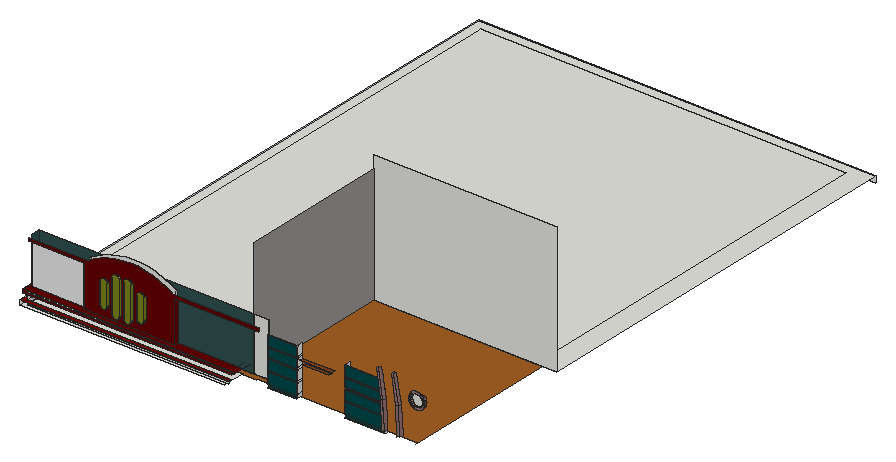
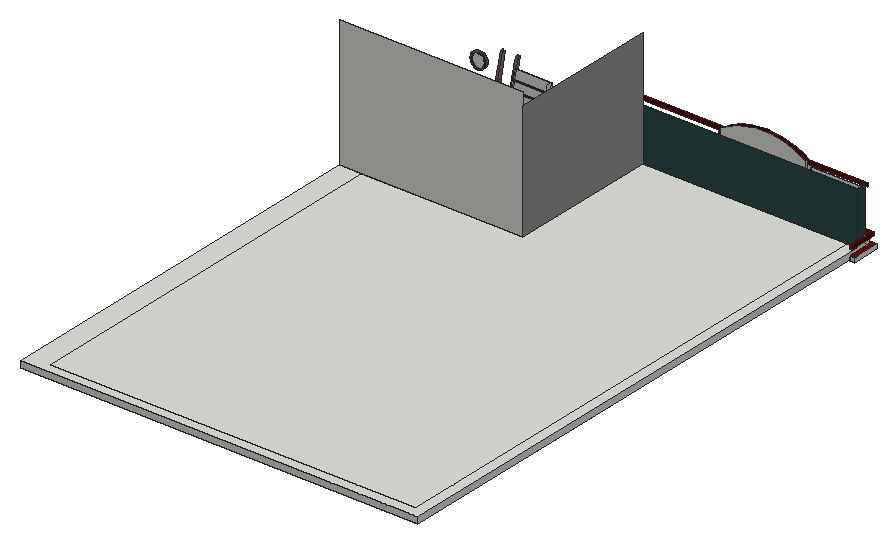
# SketchUp Ruby script. Lengths in inches.
U = 1.inch
M = Sketchup.active_model
def pt(a) = Geom::Point3d.new(a.map { |v| v * U })
def face(e, loops, mat)
  f = e.add_face(loops[0].map { |a| pt(a) })
  loops[1..].each { |l| e.add_face(l.map { |a| pt(a) }).erase! }
  f.material = f.back_material = mat if mat
  f
end
# faces: each face lists its corners as indices into pts; further lists are holes
def faces(e, pts, list, mat = nil) = list.each { |f| face(e, (f[0].is_a?(Array) ? f : [f]).map { |l| l.map { |i| pts[i] } }, mat) }
# xy, xz, yz: faces in a plane at the given z, y or x. An outline is a flat list of corners, or four numbers for a rectangle; further outlines are holes
def ring(l) = l.size == 4 ? [[l[0], l[1]], [l[2], l[1]], [l[2], l[3]], [l[0], l[3]]] : l.each_slice(2).to_a
def flat(e, list, mat, &to3) = list.each { |f| face(e, (f[0].is_a?(Array) ? f : [f]).map { |l| ring(l).map { |u, v| to3.(u, v) } }, mat) }
def xy(e, z, list, mat = nil) = flat(e, list, mat) { |x, y| [x, y, z] }
def xz(e, y, list, mat = nil) = flat(e, list, mat) { |x, z| [x, y, z] }
def yz(e, x, list, mat = nil) = flat(e, list, mat) { |y, z| [x, y, z] }
def lines(e, pts, list) = list.each { |a, b| e.add_line(pt(pts[a]), pt(pts[b])) }
# prism: a flat outline (further loops are holes) pulled along v
def prism(e, loops, v, mat = nil)
  f = face(e, loops, mat); d = Geom::Vector3d.new(v.map { |x| x * U })
  f.pushpull(f.normal.samedirection?(d) ? d.length : -d.length)
end
def box(e, o, s, mat = nil) = prism(e, [[o, [o[0] + s[0], o[1], o[2]], [o[0] + s[0], o[1] + s[1], o[2]], [o[0], o[1] + s[1], o[2]]]], [0, 0, s[2]], mat)
def at(x, y, z, deg = 0) = Geom::Transformation.translation(pt([x, y, z])) * Geom::Transformation.rotation(ORIGIN, Z_AXIS, deg.degrees)
def axes(o, x, y, z) = Geom::Transformation.new([*x, 0, *y, 0, *z, 0, *pt(o).to_a, 1])
def part(name) = M.definitions.add(name)
# library, detail: a bought-in or finely detailed component or shape, given as its bounding box
def library(name, o, s) = part(name).tap { |d| box(d.entities, o, s) }
def detail(e, o, s) = box(e.add_group.entities, o, s)
def put(e, d, t, mat = nil) = e.add_instance(d, t).tap { |i| i.material = mat if mat }
def group(e, t, mat = nil) = e.add_group.tap { |g| g.transformation = t; g.material = mat if mat }.entities
root = M.entities
M.materials.add("[0001_PaleVioletRed]").color = [219, 112, 147]
M.materials.add("[0022_Maroon]").color = [99, 0, 0]
M.materials.add("[0022_Maroon]1").color = [128, 0, 0]
M.materials.add("[0043_SaddleBrown]").color = [139, 69, 19]
M.materials.add("[0057_DarkKhaki]").color = [122, 132, 27]
M.materials.add("[0078_DarkSlateGray]").color = [47, 79, 79]
M.materials.add("[0119_RosyBrown]").color = [150, 114, 114]
M.materials.add("[Color H08]").color = [0, 71, 71]
M.materials.add("[Concrete Aggregate Smoke]").color = [154, 150, 148]
M.materials.add("[Polished Concrete Old]").color = [229, 229, 229]
M.materials.add("[Wood Square Tile 02]").color = [160, 95, 34]
xy(root,244.39,[[2.625,634.61,2.625,660.18,7.28,660.18,7.28,637.61,193.58,637.61,193.58,634.61]])
xy(root,245.03,[[221.0625,650.11,247.97,651.11],[292.45,650.11,328.99,651.11]],"[Color H08]")
xy(root,245.51,[[7,637.61,7.28,654.03],[7.28,637.61,194.39,654.03],[7,654.03,7.28,654.11],[7,654.11,7.28,660.18],[7.28,654.11,29.57,654.11,29.57,663.11,7,663.11,7,660.18,7.28,660.18],
  [[71.2,714.73,131.64,714.73,131.64,851.92,121.29,851.92,121.29,841.18,126.31,841.18,126.31,725.47,76.53,725.47,76.53,779.39,114.56,779.39,114.56,851.92,71.2,851.92],[76.53,788.7,109.94,841.18]],[7,756.4375,11.62,787.78],[11.62,756.4375,16,787.78],[7,927.36,358,927.36,358,933.36,16,933.36,16,1154.11,358,1154.11,358,1163.11,7,1163.11]])
xy(root,245.51,[[[25.34,691.07,164.1,890.37],[71.2,714.73,131.64,714.73,131.64,851.92,121.29,851.92,121.29,841.18,126.31,841.18,126.31,725.47,76.53,725.47,76.53,779.39,114.56,779.39,114.56,851.92,71.2,851.92]],[76.53,788.7,109.94,841.18]],"[0057_DarkKhaki]")
xy(root,245.51,[[[7.28,654.03,7.28,654.11,29.57,654.11,29.57,663.11,7,663.11,7,1163.11,358,1163.11,358,654.11,207.9375,654.11,207.9375,654.03],[11.62,663.42,177.82,918.03]]],"[Wood Square Tile 02]")
xy(root,247.73,[[221.0625,650.11,247.97,651.11],[292.45,650.11,329.17,651.11]],"[Color H08]")
xy(root,247.85,[[[11.62,663.42,177.82,918.03],[25.34,691.07,164.1,890.37]]],"[0001_PaleVioletRed]")
xy(root,248.7,[[2.625,634.61,197.0625,634.61,197.0625,637.61,7,637.61,7,660.18,2.625,660.18]],"[0022_Maroon]1")
xy(root,251.36,[[207.9375,651.11,221.0625,651.24],[7,651.24,16,651.24,16,1154.11,358,1154.11,358,791.05,377.9375,791.05,377.9375,1163.11,7,1163.11],[16,651.24,207,651.24,207,791.05,358,791.05,358,1154.11,16,1154.11]])
xy(root,254.68,[[4.6875,634.61,4.6875,660.18,7,660.18,7,637.61,200.08,637.61,200.08,634.61]],"[0022_Maroon]")
xy(root,258.06,[[57.84,639.11,143.09,640.93],[57.84,640.93,57.84,642.11,61.4,642.11,61.4,643.36,141.15,643.36,141.15,642.11,143.09,642.11,143.09,640.93]])
xy(root,258.06,[[4.6875,634.61,203.6875,634.61,203.6875,642.11,143.09,642.11,143.09,639.11,57.84,639.11,57.84,642.11,7,642.11,7,660.18,4.6875,660.18]],"[0022_Maroon]")
xy(root,258.11,[[221.0625,650.11,247.97,651.11],[292.45,650.11,328.77,651.11]],"[Color H08]")
xy(root,259.56,[[221.0625,650.11,247.97,651.11],[292.45,650.11,328.72,651.11]],"[Color H08]")
xy(root,268.56,[[221.0625,650.11,247.97,651.11],[292.45,650.11,328.375,651.11]],"[Color H08]")
xy(root,270.44,[[221.0625,650.11,247.97,651.11],[292.45,650.11,328.3,651.11]],"[Color H08]")
xy(root,278.01,[[221.0625,650.11,247.97,651.11],[292.45,650.11,327.36,651.11]],"[Color H08]")
xy(root,278.93,[[258.01,645.11,281.88,648.11]],"[0043_SaddleBrown]")
xy(root,279.73,[[221.0625,650.11,247.97,651.11],[292.45,650.11,327.07,651.11]],"[Color H08]")
xy(root,281.93,[[255.01,645.11,284.88,648.11]],"[0043_SaddleBrown]")
xz(root,637.11,[[89.45,261.33,90.33,261.4375,91.15,261.74,91.89,262.23,92.49,262.875,92.93,263.64,93.17,264.49,93.17,295.18,92.89,295.99,92.44,296.72,91.84,297.33,91.12,297.79,90.31,298.08,89.45,298.18,88.6,298.08,87.79,297.79,87.0625,297.33,86.46,296.72,86.01,295.99,85.73,295.18,85.73,264.49,85.98,263.64,86.41,262.875,87.01,262.23,87.75,261.74,88.58,261.4375],[100.39,261.33,101.26,261.4375,102.09,261.74,102.83,262.23,103.43,262.875,103.86,263.64,104.11,264.49,104.11,295.18,103.83,295.99,103.38,296.72,102.78,297.33,102.05,297.79,101.24,298.08,100.39,298.18,99.54,298.08,98.73,297.79,98,297.33,97.4,296.72,96.95,295.99,96.67,295.18,96.67,264.49,96.91,263.64,97.35,262.875,97.95,262.23,98.6875,261.74,99.51,261.4375],[78.26,265.89,79.12,266.01,79.92,266.34,80.6,266.86,81.13,267.55,81.46,268.35,81.57,269.21,81.57,288.64,81.27,289.31,80.85,289.9,80.31,290.38,79.67,290.75,78.98,290.97,78.26,291.05,77.54,290.97,76.84,290.75,76.21,290.38,75.67,289.9,75.24,289.31,74.95,288.64,74.95,269.21,75.06,268.35,75.39,267.55,75.92,266.86,76.6,266.34,77.4,266.01],[112.38,265.89,113.24,266.01,114.04,266.34,114.73,266.86,115.25,267.55,115.58,268.35,115.7,269.21,115.7,288.64,115.4,289.31,114.97,289.9,114.43,290.38,113.8,290.75,113.11,290.97,112.38,291.05,111.66,290.97,110.97,290.75,110.34,290.38,109.8,289.9,109.37,289.31,109.07,288.64,109.07,269.21,109.18,268.35,109.52,267.55,110.04,266.86,110.73,266.34,111.53,266.01]],"[0057_DarkKhaki]")
xz(root,637.61,[[7.28,244.39,194.39,245.51],[7,245.51,7.28,248.7]])
xz(root,639.11,[[[57.84,258.06,143.09,258.06,143.09,296.25,221.0625,296.25,221.0625,299.9,140.36,299.9,140.36,300.29,134.72,303.6,128.42,306.52,121.85,308.82,115.1,310.48,108.22,311.49,101.28,311.82,94.33,311.49,87.45,310.48,80.7,308.82,74.14,306.52,67.83,303.6,61.62,299.95,7,299.95,7,296.97,57.84,296.97],[89.45,261.33,88.58,261.4375,87.75,261.74,87.01,262.23,86.41,262.875,85.98,263.64,85.73,264.49,85.73,295.18,86.01,295.99,86.46,296.72,87.0625,297.33,87.79,297.79,88.6,298.08,89.45,298.18,90.31,298.08,91.12,297.79,91.84,297.33,92.44,296.72,92.89,295.99,93.17,295.18,93.17,264.49,92.93,263.64,92.49,262.875,91.89,262.23,91.15,261.74,90.33,261.4375],[100.39,261.33,99.51,261.4375,98.6875,261.74,97.95,262.23,97.35,262.875,96.91,263.64,96.67,264.49,96.67,295.18,96.95,295.99,97.4,296.72,98,297.33,98.73,297.79,99.54,298.08,100.39,298.18,101.24,298.08,102.05,297.79,102.78,297.33,103.38,296.72,103.83,295.99,104.11,295.18,104.11,264.49,103.86,263.64,103.43,262.875,102.83,262.23,102.09,261.74,101.26,261.4375],[78.26,265.89,77.4,266.01,76.6,266.34,75.92,266.86,75.39,267.55,75.06,268.35,74.95,269.21,74.95,288.64,75.24,289.31,75.67,289.9,76.21,290.38,76.84,290.75,77.54,290.97,78.26,291.05,78.98,290.97,79.67,290.75,80.31,290.38,80.85,289.9,81.27,289.31,81.57,288.64,81.57,269.21,81.46,268.35,81.13,267.55,80.6,266.86,79.92,266.34,79.12,266.01],[112.38,265.89,111.53,266.01,110.73,266.34,110.04,266.86,109.52,267.55,109.18,268.35,109.07,269.21,109.07,288.64,109.37,289.31,109.8,289.9,110.34,290.38,110.97,290.75,111.66,290.97,112.38,291.05,113.11,290.97,113.8,290.75,114.43,290.38,114.97,289.9,115.4,289.31,115.7,288.64,115.7,269.21,115.58,268.35,115.25,267.55,114.73,266.86,114.04,266.34,113.24,266.01]]],"[0022_Maroon]")
xz(root,642.11,[[57.84,258.06,61.4,298.09],[141.15,258.06,143.09,296.25]])
xz(root,642.11,[[7,258.06,57.84,296.97]],"[Polished Concrete Old]")
xz(root,643.36,[[61.4,258.06,61.4,300.74,67.46,304.29,73.84,307.25,80.47,309.58,87.3,311.26,94.26,312.27,101.28,312.61,108.3,312.27,115.25,311.26,122.08,309.58,128.71,307.25,135.09,304.29,141.15,300.74,141.15,258.06]])
xz(root,649.11,[[[360.63,275.86,362.59,276.11,364.42,276.87,365.98,278.07,367.18,279.64,367.94,281.46,368.2,283.42,367.94,285.375,367.18,287.2,365.98,288.77,364.42,289.97,362.59,290.72,360.63,290.98,358.68,290.72,356.85,289.97,355.29,288.77,354.09,287.2,353.33,285.375,353.07,283.42,353.33,281.46,354.09,279.64,355.29,278.07,356.85,276.87,358.68,276.11],[360.63,277.52,359.11,277.72,357.6875,278.3125,356.47,279.25,355.53,280.47,354.94,281.89,354.74,283.42,354.94,284.94,355.53,286.37,356.47,287.59,357.6875,288.52,359.11,289.11,360.63,289.3125,362.16,289.11,363.58,288.52,364.8,287.59,365.74,286.37,366.33,284.94,366.53,283.42,366.33,281.89,365.74,280.47,364.8,279.25,363.58,278.3125,362.16,277.72]]],"[0119_RosyBrown]")
xz(root,650.11,[[221.0625,247.73,247.97,258.11],[292.45,247.73,329.17,247.73,328.77,258.11,292.45,258.11],[221.0625,259.56,247.97,268.56],[292.45,259.56,328.72,259.56,328.375,268.56,292.45,268.56],[221.0625,270.44,247.97,278.01],
  [292.45,270.44,328.3,270.44,328.2,273.08,327.36,278.01,292.45,278.01],[221.0625,279.73,247.97,288.67],[292.45,279.73,327.07,279.73,325.55,288.67,292.45,288.67]],"[Color H08]")
xz(root,651.11,[[328.99,245.03,331.29,245.03,331.5,247.73,329.17,247.73,329.19,247.23],[221.0625,247.73,247.97,258.11],[292.45,247.73,292.45,258.11,328.77,258.11,329.17,247.73],[329.17,247.73,331.5,247.73,331.53,248.09,331.03,258.11,328.77,258.11],[328.77,258.11,331.03,258.11,330.96,259.56,328.72,259.56],
  [221.0625,259.56,247.97,268.56],[292.45,259.56,292.45,268.56,328.375,268.56,328.72,259.56],[328.72,259.56,330.96,259.56,330.5,268.56,328.375,268.56],[328.375,268.56,330.5,268.56,330.41,270.44,328.3,270.44],[221.0625,270.44,247.97,278.01],
  [292.45,270.44,292.45,278.01,327.36,278.01,328.2,273.08,328.3,270.44],[328.3,270.44,330.41,270.44,330.25,273.68,329.47,278.01,327.36,278.01,328.2,273.08],[360.63,277.52,362.16,277.72,363.58,278.3125,364.8,279.25,365.74,280.47,366.33,281.89,366.53,283.42,366.33,284.94,365.74,286.37,364.8,287.59,363.58,288.52,362.16,289.11,360.63,289.3125,359.11,289.11,357.6875,288.52,356.47,287.59,355.53,286.37,354.94,284.94,354.74,283.42,354.94,281.89,355.53,280.47,356.47,279.25,357.6875,278.3125,359.11,277.72],[327.36,278.01,329.47,278.01,329.16,279.73,327.07,279.73],[221.0625,279.73,247.97,288.67],
  [292.45,279.73,292.45,288.67,325.55,288.67,327.07,279.73],[327.07,279.73,329.16,279.73,327.54,288.67,325.55,288.67]])
xz(root,651.11,[[221.0625,245.03,247.97,247.73],[292.45,245.03,328.99,245.03,329.19,247.23,329.17,247.73,292.45,247.73],[221.0625,258.11,247.97,259.56],[292.45,258.11,328.77,258.11,328.72,259.56,292.45,259.56],[221.0625,268.56,247.97,270.44],
  [292.45,268.56,328.375,268.56,328.3,270.44,292.45,270.44],[221.0625,278.01,247.97,279.73],[292.45,278.01,327.36,278.01,327.07,279.73,292.45,279.73]],"[Color H08]")
xz(root,651.24,[[207,251.36,221.0625,300.74]])
xz(root,651.24,[[7,251.36,207,300.74]],"[0078_DarkSlateGray]")
xz(root,660.18,[[2.625,244.39,2.625,248.7,7,248.7,7,245.51,7.28,245.51,7.28,244.39]])
xz(root,660.18,[[4.6875,254.68,7,258.06]],"[0022_Maroon]")
xz(root,663.42,[[11.62,245.51,177.82,247.85]],"[0001_PaleVioletRed]")
xz(root,691.07,[[25.34,245.51,164.1,247.85]],"[0057_DarkKhaki]")
xz(root,791.05,[[207,251.36,377.9375,372.74]])
xz(root,890.37,[[25.34,245.51,164.1,247.85]],"[0057_DarkKhaki]")
xz(root,918.03,[[11.62,245.51,177.82,247.85]])
xz(root,1163.11,[[7,245.51,377.9375,251.36]])
yz(root,2.625,[[634.61,244.39,660.18,248.7]])
yz(root,4.6875,[[634.61,254.68,660.18,258.06]],"[0022_Maroon]")
yz(root,7,[[637.61,245.51,654.11,248.7],[654.11,245.51,660.18,248.7],[642.11,254.68,651.24,258.06],[651.24,254.68,660.18,258.06]])
yz(root,7,[[642.11,258.06,651.24,300.74]],"[0078_DarkSlateGray]")
yz(root,7,[[660.18,245.51,660.18,248.7,637.61,248.7,637.61,254.68,651.24,254.68,651.24,251.36,1163.11,251.36,1163.11,245.51]],"[Polished Concrete Old]")
yz(root,7.28,[[637.61,244.39,660.18,245.51]])
yz(root,11.62,[[663.42,245.51,741.9,247.85],[741.9,245.51,918.03,247.85]],"[0001_PaleVioletRed]")
yz(root,25.34,[[691.07,245.51,741.9,247.85],[741.9,245.51,890.37,247.85]],"[0057_DarkKhaki]")
yz(root,57.84,[[639.11,258.06,642.11,296.97]],"[0022_Maroon]")
yz(root,61.4,[[642.11,258.06,643.36,300.61]])
yz(root,74.95,[[637.11,269.21,639.11,288.64]],"[0057_DarkKhaki]")
yz(root,81.57,[[637.11,269.21,639.11,288.64]],"[0057_DarkKhaki]")
yz(root,85.73,[[637.11,264.49,639.11,295.18]],"[0057_DarkKhaki]")
yz(root,93.17,[[637.11,264.49,639.11,295.18]],"[0057_DarkKhaki]")
yz(root,96.67,[[637.11,264.49,639.11,295.18]],"[0057_DarkKhaki]")
yz(root,104.11,[[637.11,264.49,639.11,295.18]],"[0057_DarkKhaki]")
yz(root,109.07,[[637.11,269.21,639.11,288.64]],"[0057_DarkKhaki]")
yz(root,115.7,[[637.11,269.21,639.11,288.64]],"[0057_DarkKhaki]")
yz(root,141.15,[[642.11,258.06,643.36,300.67]])
yz(root,143.09,[[639.11,258.06,642.11,296.25]],"[0022_Maroon]")
yz(root,164.1,[[691.07,245.51,890.37,247.85]],"[0057_DarkKhaki]")
yz(root,177.82,[[663.42,245.51,918.03,247.85]],"[0001_PaleVioletRed]")
yz(root,207,[[651.24,251.36,791.05,360.74]],"[Concrete Aggregate Smoke]")
yz(root,221.0625,[[650.11,247.73,651.11,251.36],[650.11,251.36,651.11,258.11],[651.11,251.36,651.24,300.74],[650.11,259.56,651.11,268.56],[650.11,270.44,651.11,278.01],
  [650.11,279.73,651.11,288.67]])
yz(root,247.97,[[651.11,245.03,656.36,247.73],[650.11,247.73,651.11,258.11],[651.11,247.73,656.36,258.11],[651.11,258.11,656.36,259.56],[650.11,259.56,651.11,268.56],
  [651.11,259.56,656.36,268.56],[651.11,268.56,656.36,270.44],[650.11,270.44,651.11,278.01],[651.11,270.44,656.36,278.01],[651.11,278.01,656.36,279.73],
  [650.11,279.73,651.11,288.67],[651.11,279.73,656.36,288.67]])
yz(root,292.45,[[651.11,245.03,656.36,247.73],[650.11,247.73,651.11,258.11],[651.11,247.73,656.36,258.11],[651.11,258.11,656.36,259.56],[650.11,259.56,651.11,268.56],
  [651.11,259.56,656.36,268.56],[651.11,268.56,656.36,270.44],[650.11,270.44,651.11,278.01],[651.11,270.44,656.36,278.01],[651.11,278.01,656.36,279.73],
  [650.11,279.73,651.11,288.67],[651.11,279.73,656.36,288.67]])
p = [[329.17,651.11,247.73],[329.19,651.11,247.23],[329.19,648.11,247.23],[328.2,648.11,273.08],[328.2,650.11,273.08],[328.3,650.11,270.44],
  [328.3,651.11,270.44],[328.375,651.11,268.56],[328.375,650.11,268.56],[328.72,650.11,259.56],[328.72,651.11,259.56],[328.77,651.11,258.11],
  [328.77,650.11,258.11],[329.17,650.11,247.73],[342.28,651.11,273.08],[343.27,651.11,247.23],[343.27,648.11,247.23],[342.28,648.11,273.08],
  [331.53,651.11,248.09],[331.03,651.11,258.11],[330.96,651.11,259.56],[330.5,651.11,268.56],[330.41,651.11,270.44],[330.25,651.11,273.68],
  [330.25,648.11,273.68],[331.53,648.11,248.09],[345.61,651.11,248.09],[344.33,651.11,273.68],[344.33,648.11,273.68],[345.61,648.11,248.09],
  [88.58,639.11,261.4375],[89.45,639.11,261.33],[89.45,637.11,261.33],[88.58,637.11,261.4375],[90.33,639.11,261.4375],[90.33,637.11,261.4375],
  [99.51,639.11,261.4375],[100.39,639.11,261.33],[100.39,637.11,261.33],[99.51,637.11,261.4375],[101.26,639.11,261.4375],[101.26,637.11,261.4375],
  [87.75,639.11,261.74],[87.75,637.11,261.74],[91.15,639.11,261.74],[91.15,637.11,261.74],[98.6875,639.11,261.74],[98.6875,637.11,261.74],
  [102.09,639.11,261.74],[102.09,637.11,261.74],[87.01,639.11,262.23],[87.01,637.11,262.23],[91.89,639.11,262.23],[91.89,637.11,262.23],
  [97.95,639.11,262.23],[97.95,637.11,262.23],[102.83,639.11,262.23],[102.83,637.11,262.23],[86.41,639.11,262.875],[86.41,637.11,262.875],
  [92.49,639.11,262.875],[92.49,637.11,262.875],[97.35,639.11,262.875],[97.35,637.11,262.875],[103.43,639.11,262.875],[103.43,637.11,262.875],
  [85.98,639.11,263.64],[85.98,637.11,263.64],[92.93,639.11,263.64],[92.93,637.11,263.64],[96.91,639.11,263.64],[96.91,637.11,263.64],
  [103.86,639.11,263.64],[103.86,637.11,263.64],[85.73,639.11,264.49],[85.73,637.11,264.49],[93.17,639.11,264.49],[93.17,637.11,264.49],
  [96.67,639.11,264.49],[96.67,637.11,264.49],[104.11,639.11,264.49],[104.11,637.11,264.49],[77.4,639.11,266.01],[78.26,639.11,265.89],
  [78.26,637.11,265.89],[77.4,637.11,266.01],[79.12,639.11,266.01],[79.12,637.11,266.01],[111.53,639.11,266.01],[112.38,639.11,265.89],
  [112.38,637.11,265.89],[111.53,637.11,266.01],[113.24,639.11,266.01],[113.24,637.11,266.01],[76.6,639.11,266.34],[76.6,637.11,266.34],
  [79.92,639.11,266.34],[79.92,637.11,266.34],[110.73,639.11,266.34],[110.73,637.11,266.34],[114.04,639.11,266.34],[114.04,637.11,266.34],
  [75.92,639.11,266.86],[75.92,637.11,266.86],[80.6,639.11,266.86],[80.6,637.11,266.86],[110.04,639.11,266.86],[110.04,637.11,266.86],
  [114.73,639.11,266.86],[114.73,637.11,266.86],[75.39,639.11,267.55],[75.39,637.11,267.55],[81.13,639.11,267.55],[81.13,637.11,267.55],
  [109.52,639.11,267.55],[109.52,637.11,267.55],[115.25,639.11,267.55],[115.25,637.11,267.55],[75.06,639.11,268.35],[75.06,637.11,268.35],
  [81.46,639.11,268.35],[81.46,637.11,268.35],[109.18,639.11,268.35],[109.18,637.11,268.35],[115.58,639.11,268.35],[115.58,637.11,268.35],
  [74.95,639.11,269.21],[74.95,637.11,269.21],[81.57,639.11,269.21],[81.57,637.11,269.21],[109.07,639.11,269.21],[109.07,637.11,269.21],
  [115.7,639.11,269.21],[115.7,637.11,269.21],[328.2,651.11,273.08],[327.07,651.11,279.73],[327.36,651.11,278.01],[327.36,650.11,278.01],
  [323.87,648.11,298.58],[323.87,650.11,298.58],[325.22,650.11,290.61],[325.22,651.11,290.61],[325.55,651.11,288.67],[325.55,650.11,288.67],
  [327.07,650.11,279.73],[337.94,651.11,298.58],[337.94,648.11,298.58],[329.47,651.11,278.01],[329.16,651.11,279.73],[327.54,651.11,288.67],
  [327.19,651.11,290.61],[325.7,651.11,298.89],[325.7,648.11,298.89],[339.78,651.11,298.89],[339.78,648.11,298.89],[358.68,651.11,276.11],
  [360.63,651.11,275.86],[360.63,649.11,275.86],[358.68,649.11,276.11],[362.59,651.11,276.11],[362.59,649.11,276.11],[356.85,651.11,276.87],
  [356.85,649.11,276.87],[364.42,651.11,276.87],[364.42,649.11,276.87],[355.29,651.11,278.07],[355.29,649.11,278.07],[365.98,651.11,278.07],
  [365.98,649.11,278.07],[360.63,651.11,277.52],[359.11,651.11,277.72],[359.11,649.11,277.72],[360.63,649.11,277.52],[362.16,651.11,277.72],
  [362.16,649.11,277.72],[357.6875,651.11,278.3125],[357.6875,649.11,278.3125],[363.58,651.11,278.3125],[363.58,649.11,278.3125],[354.09,651.11,279.64],
  [354.09,649.11,279.64],[367.18,651.11,279.64],[367.18,649.11,279.64],[356.47,651.11,279.25],[356.47,649.11,279.25],[364.8,651.11,279.25],
  [364.8,649.11,279.25],[355.53,651.11,280.47],[355.53,649.11,280.47],[365.74,651.11,280.47],[365.74,649.11,280.47],[353.33,651.11,281.46],
  [353.33,649.11,281.46],[367.94,651.11,281.46],[367.94,649.11,281.46],[354.94,651.11,281.89],[354.94,649.11,281.89],[366.33,651.11,281.89],
  [366.33,649.11,281.89],[353.07,651.11,283.42],[353.07,649.11,283.42],[368.2,651.11,283.42],[368.2,649.11,283.42],[354.74,651.11,283.42],
  [354.74,649.11,283.42],[366.53,651.11,283.42],[366.53,649.11,283.42],[353.33,651.11,285.375],[353.33,649.11,285.375],[354.94,651.11,284.94],
  [354.94,649.11,284.94],[366.33,651.11,284.94],[366.33,649.11,284.94],[367.94,651.11,285.375],[367.94,649.11,285.375],[355.53,651.11,286.37],
  [355.53,649.11,286.37],[365.74,651.11,286.37],[365.74,649.11,286.37],[354.09,651.11,287.2],[354.09,649.11,287.2],[367.18,651.11,287.2],
  [367.18,649.11,287.2],[356.47,651.11,287.59],[356.47,649.11,287.59],[364.8,651.11,287.59],[364.8,649.11,287.59],[355.29,651.11,288.77],
  [355.29,649.11,288.77],[365.98,651.11,288.77],[365.98,649.11,288.77],[357.6875,651.11,288.52],[357.6875,649.11,288.52],[363.58,651.11,288.52],
  [363.58,649.11,288.52],[358,654.11,245.51],[358,651.11,245.51],[198.9375,642.11,258.06],[198.9375,651.11,258.06],[16,642.11,251.36],
  [16,642.11,258.06],[7,642.11,251.36],[16,651.24,251.36],[203.6875,642.11,258.06],[203.6875,651.11,258.06],[16,651.11,258.06]]
faces(root,p,[[0,1,2,3,4,5,6,7,8,9,10,11,12,13],[14,15,16,17],[18,19,20,21,22,23,24,25],[26,27,28,29],[135,136,137,4,3,138,139,140,141,142,143,144],[145,14,17,146],[23,147,148,149,150,151,152,24],[27,153,154,28],
  [155,156,157,158],[156,159,160,157],[161,155,158,162],[159,163,164,160],[165,161,162,166],[163,167,168,164],[169,170,171,172],[173,169,172,174],
  [170,175,176,171],[177,173,174,178],[179,165,166,180],[167,181,182,168],[175,183,184,176],[185,177,178,186],[183,187,188,184],[189,185,186,190],
  [191,179,180,192],[181,193,194,182],[187,195,196,188],[197,189,190,198],[199,191,192,200],[193,201,202,194],[195,203,204,196],[205,197,198,206],
  [207,199,200,208],[203,209,210,204],[211,205,206,212],[201,213,214,202],[209,215,216,210],[217,211,212,218],[219,207,208,220],[213,221,222,214],
  [215,223,224,216],[225,217,218,226],[227,219,220,228],[221,229,230,222],[223,231,232,224],[233,225,226,234]],"[0119_RosyBrown]")
faces(root,p,[[11,0,13,12],[7,10,9,8],[134,6,5,4],[136,134,4,137],[142,135,144,143]])
faces(root,p,[[30,31,32,33],[31,34,35,32],[36,37,38,39],[37,40,41,38],[42,30,33,43],[34,44,45,35],[46,36,39,47],[40,48,49,41],
  [50,42,43,51],[44,52,53,45],[54,46,47,55],[48,56,57,49],[58,50,51,59],[52,60,61,53],[62,54,55,63],[56,64,65,57],
  [66,58,59,67],[60,68,69,61],[70,62,63,71],[64,72,73,65],[74,66,67,75],[68,76,77,69],[78,70,71,79],[72,80,81,73],
  [82,83,84,85],[83,86,87,84],[88,89,90,91],[89,92,93,90],[94,82,85,95],[86,96,97,87],[98,88,91,99],[92,100,101,93],
  [102,94,95,103],[96,104,105,97],[106,98,99,107],[100,108,109,101],[110,102,103,111],[104,112,113,105],[114,106,107,115],[108,116,117,109],
  [118,110,111,119],[112,120,121,113],[122,114,115,123],[116,124,125,117],[126,118,119,127],[120,128,129,121],[130,122,123,131],[124,132,133,125]],"[0057_DarkKhaki]")
lines(root,p,[[235,236],[237,238],[239,240],[239,241],[242,239],[243,244],[245,240]])
